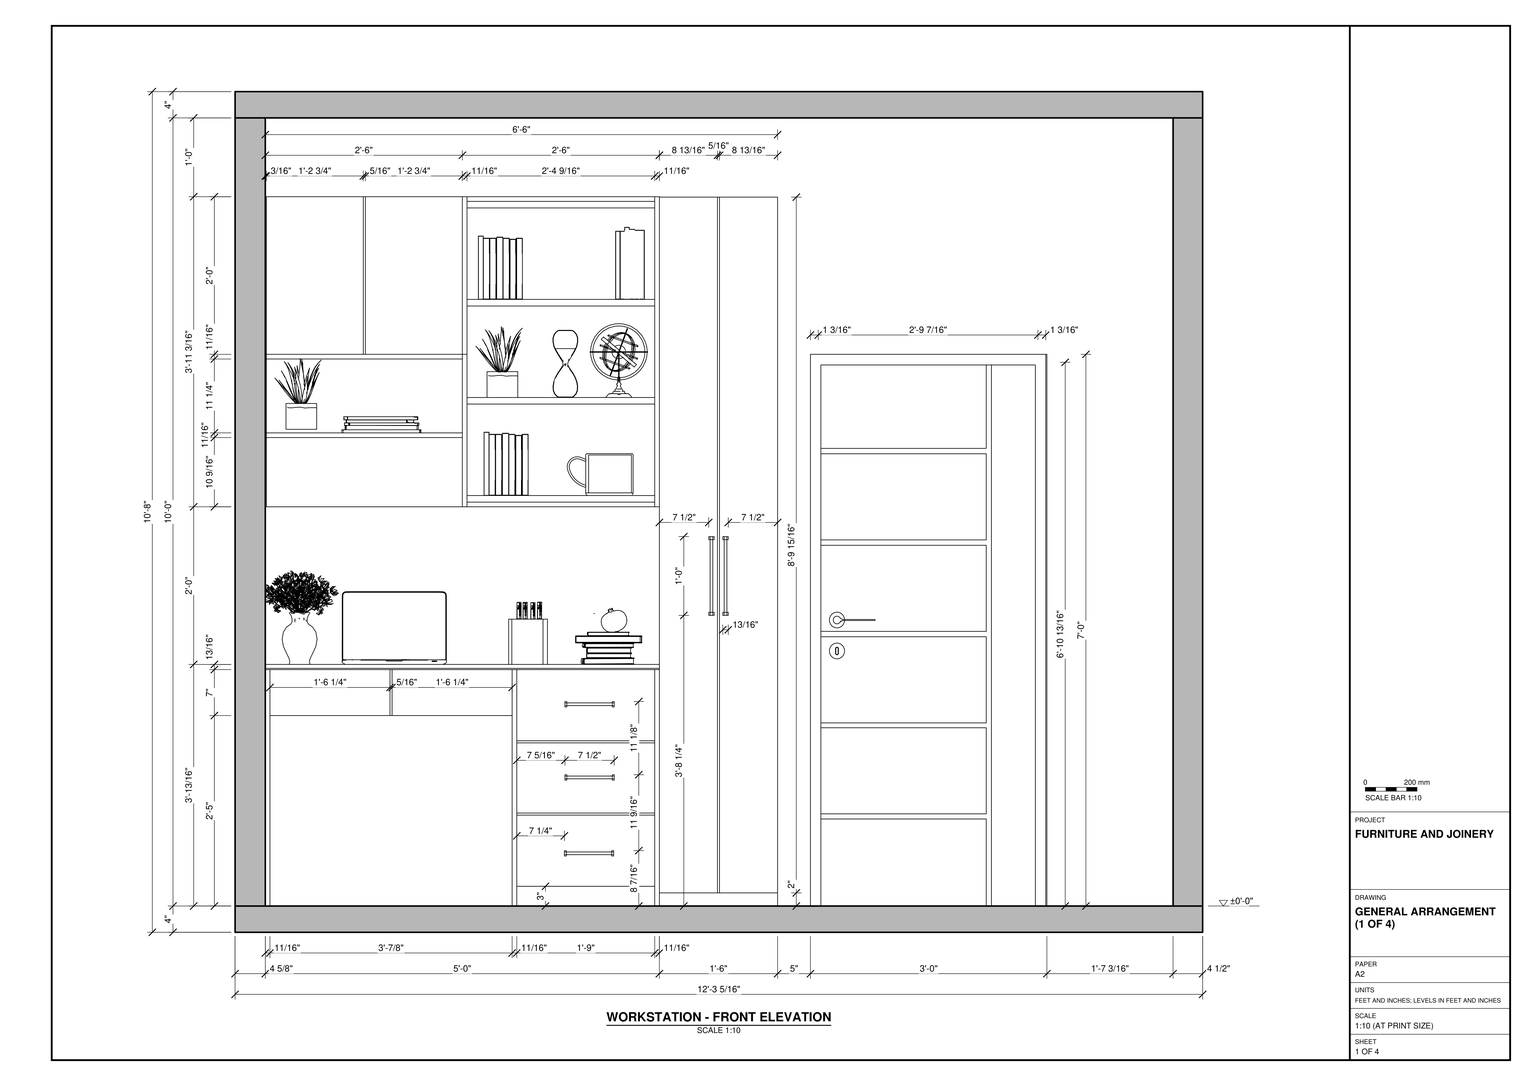
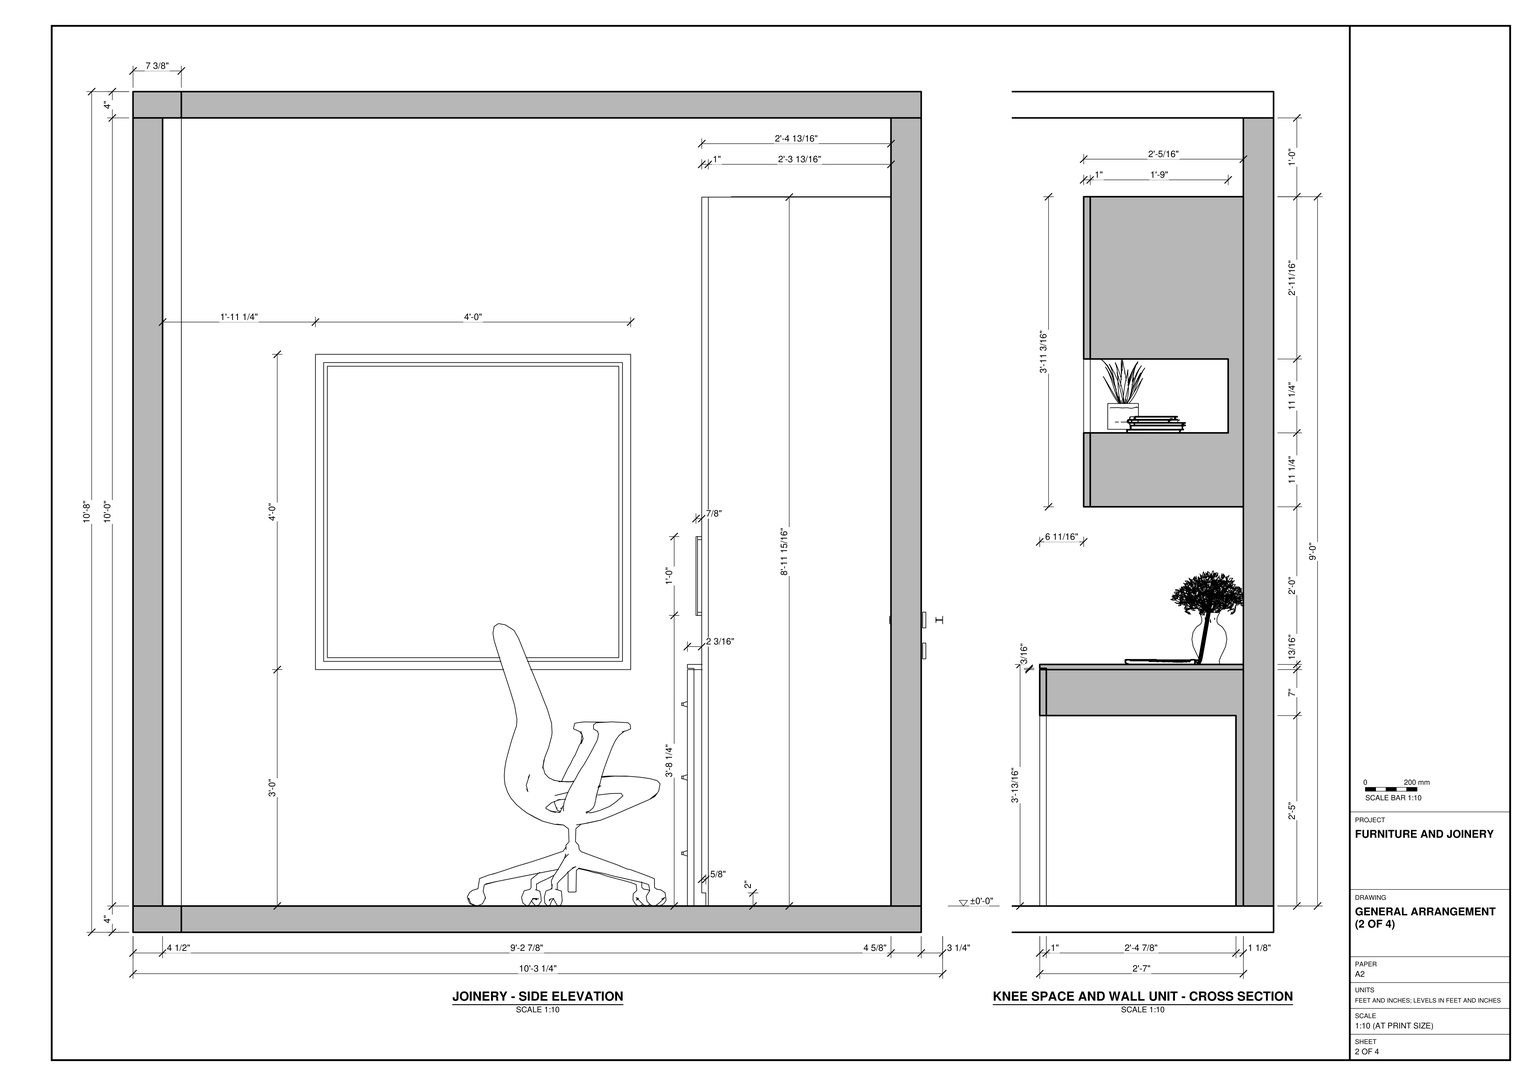
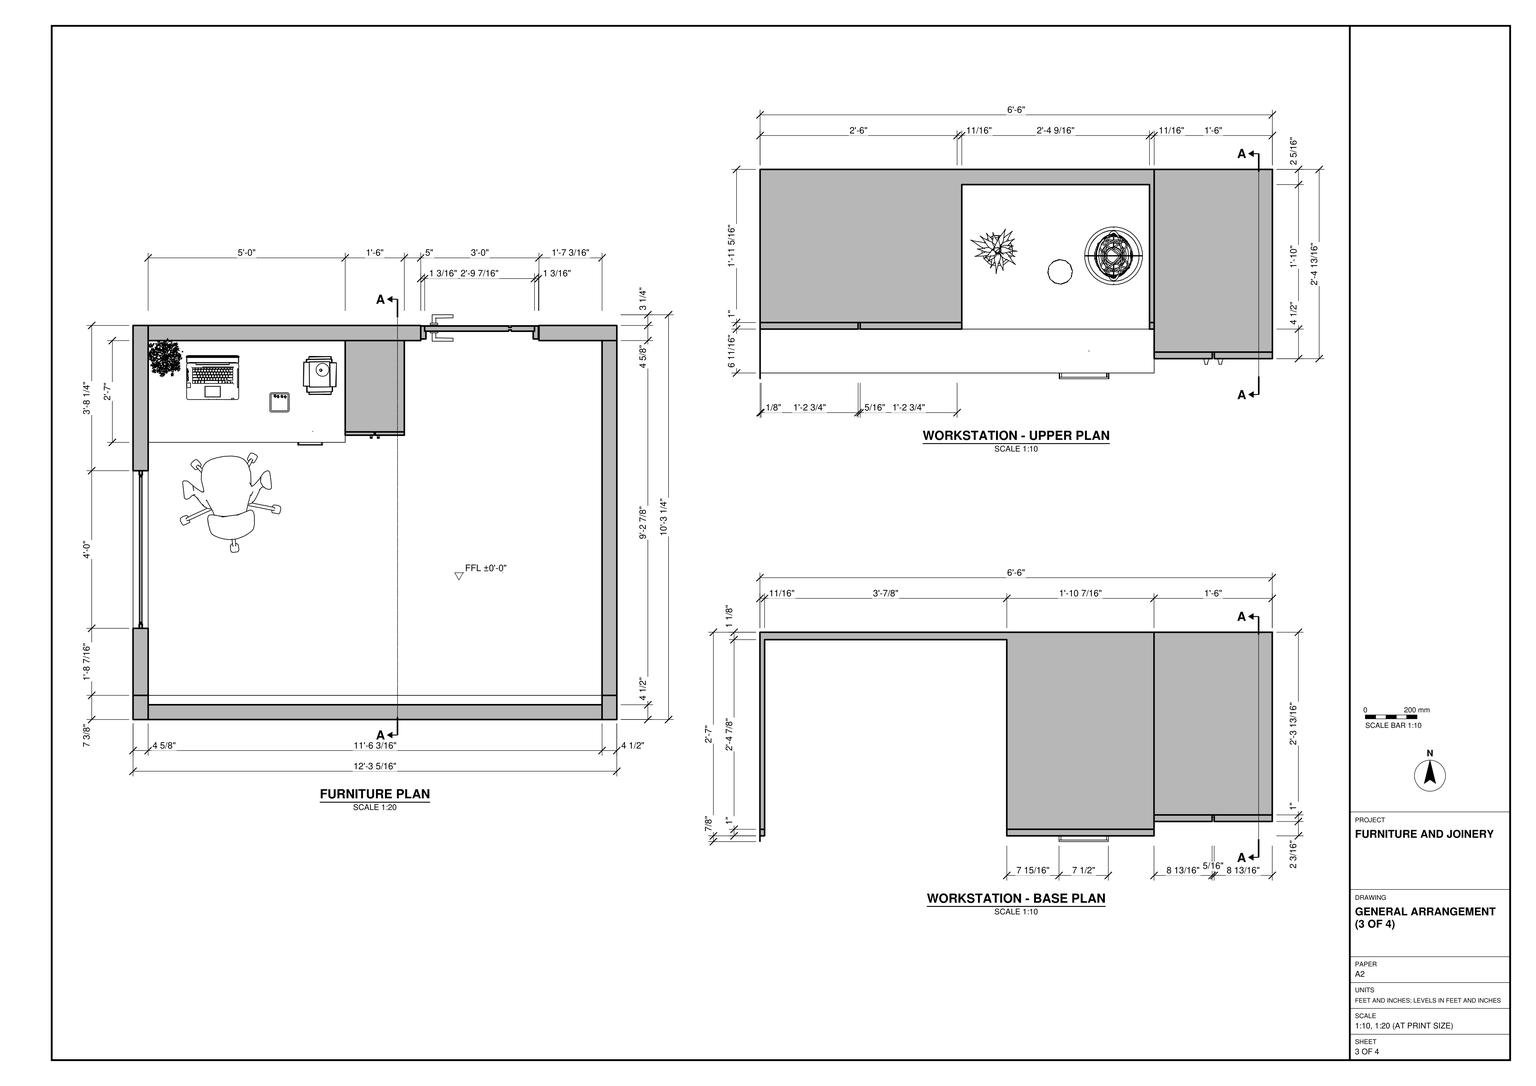
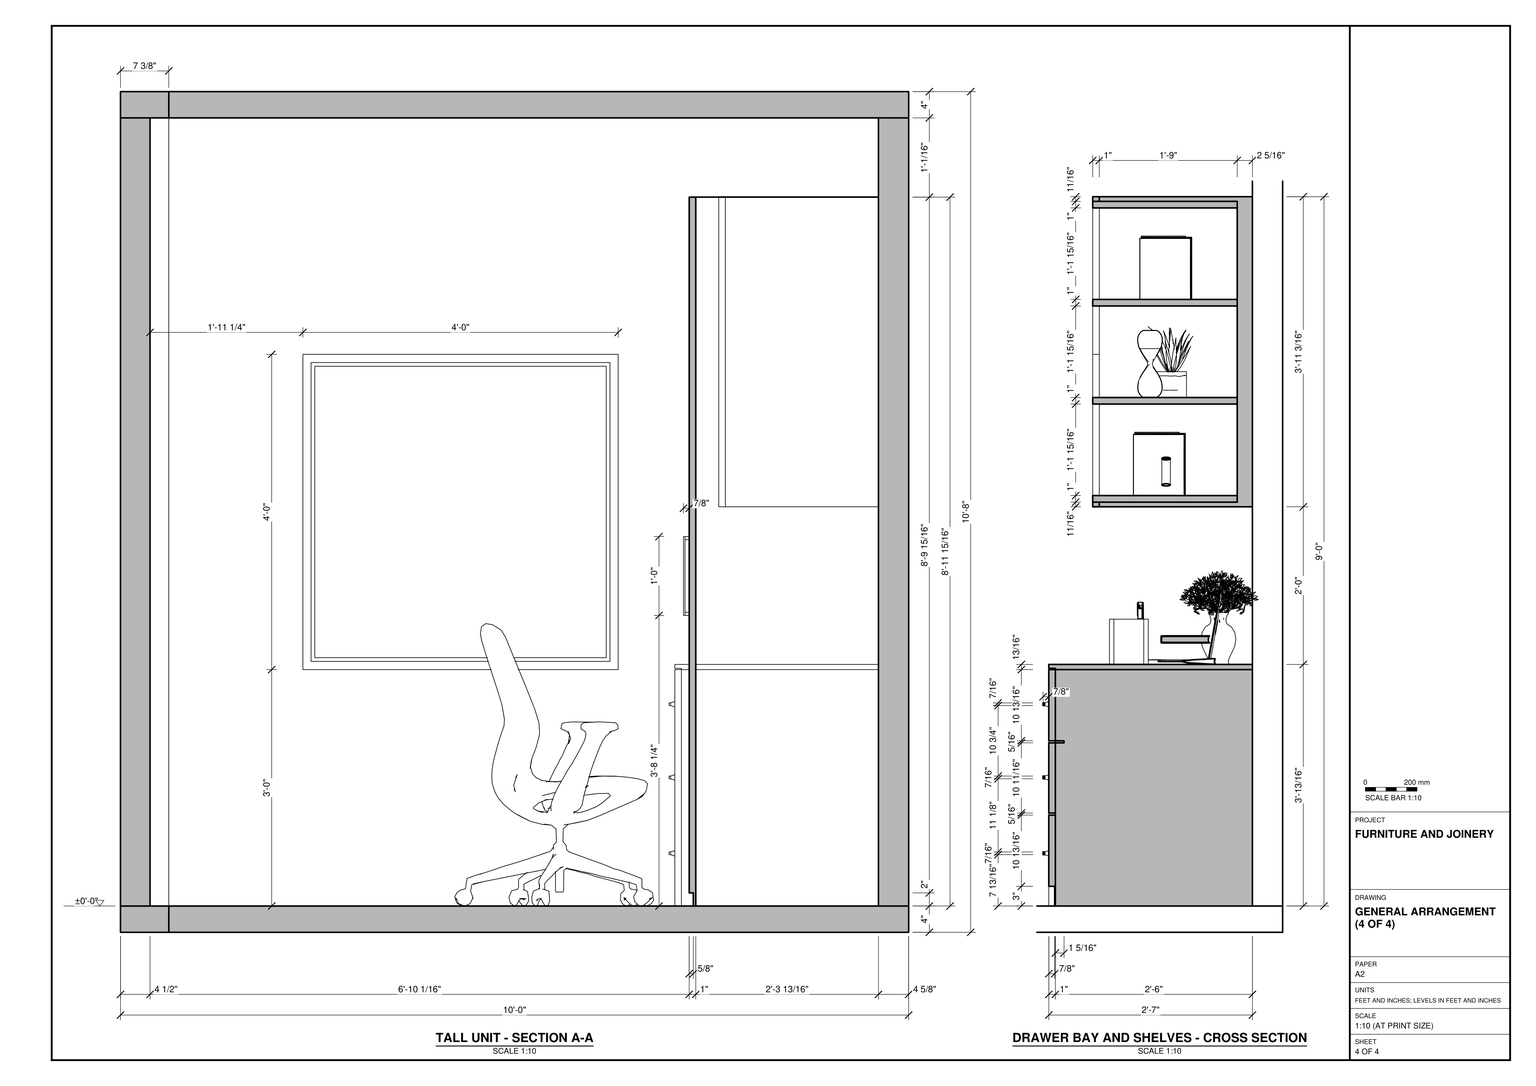
Work in feet and inches in SketchUp. Use task_files/diagram_01.pdf to model the room and its fitted workstation. The overall model measures 12'-3 5/16" along the workstation wall, 10'-3 1/4" in depth and 10'-8" in height. Set the finished floor at ±0'-0". Model the floor and ceiling slabs and follow the individual wall thicknesses in plan. Place the framed door to the right of the workstation and the square window in the adjoining left wall.

Build the workstation from the left corner toward the door. Use the base plan for the 5'-0" desk and its depth of 2'-7". Leave knee space beneath the shallow drawers and place the drawer pedestal to their right. Fit the tall paired-door cabinet between the desk and the doorway. Above the desk, reproduce the closed cupboards and open shelf bays, using the upper plan and cross section to set their depths and clearance above the worktop. Position the office chair facing the desk. Place the laptop, books, plants and desk accessories in the worktop and shelf locations shown. Decor and loose items may be any suitable library components.

Keep the walls, slabs and each furniture or joinery piece in separate groups or components, and use components for repeated parts. Save one SketchUp model as output_files/study_room_with_a_built_in_workstation.skp.

# SketchUp Ruby script. Lengths in inches.
U = 1.inch
M = Sketchup.active_model
def pt(a) = Geom::Point3d.new(a.map { |v| v * U })
def face(e, loops, mat)
  f = e.add_face(loops[0].map { |a| pt(a) })
  loops[1..].each { |l| e.add_face(l.map { |a| pt(a) }).erase! }
  f.material = f.back_material = mat if mat
  f
end
# faces: each face lists its corners as indices into pts; further lists are holes
def faces(e, pts, list, mat = nil) = list.each { |f| face(e, (f[0].is_a?(Array) ? f : [f]).map { |l| l.map { |i| pts[i] } }, mat) }
# xy, xz, yz: faces in a plane at the given z, y or x. An outline is a flat list of corners, or four numbers for a rectangle; further outlines are holes
def ring(l) = l.size == 4 ? [[l[0], l[1]], [l[2], l[1]], [l[2], l[3]], [l[0], l[3]]] : l.each_slice(2).to_a
def flat(e, list, mat, &to3) = list.each { |f| face(e, (f[0].is_a?(Array) ? f : [f]).map { |l| ring(l).map { |u, v| to3.(u, v) } }, mat) }
def xy(e, z, list, mat = nil) = flat(e, list, mat) { |x, y| [x, y, z] }
def xz(e, y, list, mat = nil) = flat(e, list, mat) { |x, z| [x, y, z] }
def yz(e, x, list, mat = nil) = flat(e, list, mat) { |y, z| [x, y, z] }
def lines(e, pts, list) = list.each { |a, b| e.add_line(pt(pts[a]), pt(pts[b])) }
# prism: a flat outline (further loops are holes) pulled along v
def prism(e, loops, v, mat = nil)
  f = face(e, loops, mat); d = Geom::Vector3d.new(v.map { |x| x * U })
  f.pushpull(f.normal.samedirection?(d) ? d.length : -d.length)
end
def box(e, o, s, mat = nil) = prism(e, [[o, [o[0] + s[0], o[1], o[2]], [o[0] + s[0], o[1] + s[1], o[2]], [o[0], o[1] + s[1], o[2]]]], [0, 0, s[2]], mat)
def at(x, y, z, deg = 0) = Geom::Transformation.translation(pt([x, y, z])) * Geom::Transformation.rotation(ORIGIN, Z_AXIS, deg.degrees)
def axes(o, x, y, z) = Geom::Transformation.new([*x, 0, *y, 0, *z, 0, *pt(o).to_a, 1])
def part(name) = M.definitions.add(name)
# library, detail: a bought-in or finely detailed component or shape, given as its bounding box
def library(name, o, s) = part(name).tap { |d| box(d.entities, o, s) }
def detail(e, o, s) = box(e.add_group.entities, o, s)
def put(e, d, t, mat = nil) = e.add_instance(d, t).tap { |i| i.material = mat if mat }
def group(e, t, mat = nil) = e.add_group.tap { |g| g.transformation = t; g.material = mat if mat }.entities
root = M.entities
M.materials.add("PVC Olive Green Matte 001").color = [133, 140, 86]
M.materials.add("Tiles Marble White 03 180cm").color = [241, 241, 241]
M.materials.add("Wood 021 27.52cm").color = [255, 255, 255]
c1 = part("POI-E1497-320-1917\#1")
xy(c1.entities,0,[[0,0,0.29,0.83],[7.21,0,7.5,0.83]])
xy(c1.entities,0.64,[[0.29,0.21,7.21,0.62]])
xy(c1.entities,0.875,[[0,0.21,7.5,0.62]])
xz(c1.entities,0.21,[[0,0.64,7.5,0.875]])
xz(c1.entities,0.62,[[0,0.64,7.5,0.875]])
yz(c1.entities,0,[[0,0,0.21,0.64,0.21,0.875,0.62,0.875,0.62,0.64,0.83,0]])
yz(c1.entities,0.29,[[0,0,0.83,0,0.62,0.64,0.21,0.64]])
yz(c1.entities,7.21,[[0,0,0.21,0.64,0.62,0.64,0.83,0]])
yz(c1.entities,7.5,[[0,0,0.83,0,0.62,0.64,0.62,0.875,0.21,0.875,0.21,0.64]])
p = [[0,0.21,0.64],[0,0,0],[0.29,0,0],[0.29,0.21,0.64],[7.21,0.21,0.64],[7.21,0,0],
  [7.5,0,0],[7.5,0.21,0.64],[0,0.83,0],[0,0.62,0.64],[0.29,0.62,0.64],[0.29,0.83,0],
  [7.5,0.83,0],[7.5,0.62,0.64],[7.21,0.62,0.64],[7.21,0.83,0]]
faces(c1.entities,p,[[0,1,2,3],[4,5,6,7],[8,9,10,11],[12,13,14,15]])
c2 = part("Group15\#1")
p = [[0,0,0],[0,0,-10.57],[-4.61,0,-10.57],[30,-4.22,0],[-30,-4.22,0],[30,4.22,0],
  [30,0,0],[-30,4.22,0],[4.61,0,-10.57],[-30,0,0],[0,0,-17.11]]
lines(c2.entities,p,[[0,1],[1,2],[3,4],[5,6],[7,5],[1,8],[9,0],[0,6],[8,10],[4,9],[6,3],[2,10],
  [9,7]])
c3 = part("Rectangle Light")
put(c3.entities,c2,at(0,0,0))
c4 = part("Group17\#1")
p = [[0,0,0],[0,0,-5.7],[-2.29,0,-5.7],[14.92,-3.53,0],[-14.92,-3.53,0],[14.92,3.53,0],
  [14.92,0,0],[-14.92,3.53,0],[2.29,0,-5.7],[-14.92,0,0],[0,0,-9.23]]
lines(c4.entities,p,[[0,1],[1,2],[3,4],[5,6],[7,5],[1,8],[9,0],[0,6],[8,10],[4,9],[6,3],[2,10],
  [9,7]])
c5 = part("Rectangle Light\#1")
put(c5.entities,c4,at(0,0,0))
c6 = part("Group19\#1")
p = [[0,0,0],[0,0,-5.18],[-2.2,0,-5.18],[14.29,-2.48,0],[-14.29,-2.48,0],[14.29,2.48,0],
  [14.29,0,0],[-14.29,2.48,0],[2.2,0,-5.18],[-14.29,0,0],[0,0,-8.39]]
lines(c6.entities,p,[[0,1],[1,2],[3,4],[5,6],[7,5],[1,8],[9,0],[0,6],[8,10],[4,9],[6,3],[2,10],
  [9,7]])
c7 = part("Rectangle Light\#2")
put(c7.entities,c6,at(0,0,0))
c8 = part("Group21\#1")
p = [[0,0,0],[0,0,-5.25],[-2.2,0,-5.25],[14.29,-2.69,0],[-14.29,-2.69,0],[14.29,2.69,0],
  [14.29,0,0],[-14.29,2.69,0],[2.2,0,-5.25],[-14.29,0,0],[0,0,-8.49]]
lines(c8.entities,p,[[0,1],[1,2],[3,4],[5,6],[7,5],[1,8],[9,0],[0,6],[8,10],[4,9],[6,3],[2,10],
  [9,7]])
c9 = part("Rectangle Light\#3")
put(c9.entities,c8,at(0,0,0))
c10 = part("Group23\#1")
p = [[0,0,0],[0,0,-5.4],[-2.2,0,-5.4],[14.29,-3.19,0],[-14.29,-3.19,0],[14.29,3.19,0],
  [14.29,0,0],[-14.29,3.19,0],[2.2,0,-5.4],[-14.29,0,0],[0,0,-8.74]]
lines(c10.entities,p,[[0,1],[1,2],[3,4],[5,6],[7,5],[1,8],[9,0],[0,6],[8,10],[4,9],[6,3],[2,10],
  [9,7]])
c11 = part("Rectangle Light\#4")
put(c11.entities,c10,at(0,0,0))
c12 = library("Laptop 013",[-7.94,-6.65,0],[15.87,13.3,11.09])
c13 = library("Vase Flowers 26-02",[-5.76,-5.9,0],[11.73,12.02,14.27])
c14 = library("Books 155 025",[-5.0625,-5.83,0.01],[10.11,11.66,8.59])
c15 = library("Books 53-13",[-3.36,-3.97,0],[6.72,7.94,9.65])
c16 = library("Books 53-17",[-2.19,-3.6875,0],[4.38,7.37,10.99])
c17 = library("pen_stand",[0,-5.91,0],[13.07,11.82,9.49])
c18 = library("Books 193 003",[-6.07,-4.15,0],[12.06,9.04,2.47])
c19 = library("Potted Succulent 003",[-4.09,-3.62,0],[7.1,6.83,10.79])
c20 = library("Decorative Hourglass 001",[-1.06,-1.06,0.02],[2.12,2.12,5.71])
c21 = library("Armillary Sphere 37-31",[-7.11,-7.1,0],[14.21,14.18,18.13])
c22 = library("Chair 233 035",[-15.42,-13.39,-0.11],[30.84,29.38,43.01])
c23 = library("PINTU 6 YA",[0,-0.6875,0],[35.83,8.07,80.71])
c24 = library("Group\#29",[0,0,0],[5.48,3.93,3.49])
c25 = part("Group88\#1")
xz(c25.entities,32.25,[[29.52,0,176.83,4]])
c26 = part("Group90\#1")
xz(c26.entities,32.25,[[29.52,4,34.12,124]])
c27 = part("Group188\#1")
xz(c27.entities,32.25,[[172.33,4,176.83,124]])
c28 = part("Group218\#1")
xz(c28.entities,32.25,[[29.52,124,176.83,128]])
c29 = part("Group83\#1")
put(c29.entities,c25,at(0,0,0))
put(c29.entities,c26,at(0,0,0))
put(c29.entities,c27,at(0,0,0))
put(c29.entities,c28,at(0,0,0))
p = [[2.3,75.77,40],[2.3,27.77,40],[2.3,27.77,88],[2.3,75.77,88]]
lines(root,p,[[0,1],[1,2],[2,3],[3,0]])
put(root,c1,axes([57.72,84.4,34.31],[-1,0,0],[0,0,1],[0,-1,0]))
put(root,c1,axes([57.72,84.4,23.17],[-1,0,0],[0,0,1],[0,-1,0]))
put(root,c1,axes([57.64,84.4,11.61],[-1,0,0],[0,0,1],[0,-1,0]))
put(root,c1,axes([72.11,86.59,48.25],[0,0,1.6],[1,0,0],[0,-1,0]))
put(root,c1,axes([74.26,86.59,48.25],[0,0,1.6],[1,0,0],[0,-1,0]))
put(root,c3,axes([34.6,111.18,64.78],[1,0,0],[0,-1,0],[0,0,0.21]))
put(root,c5,axes([19.68,109.56,87.28],[1,0,0],[0,-1,0],[0,0,0.2]))
put(root,c7,axes([49.6,110.61,110.28],[1,0,0],[0,-1,0],[0,0,0.32]))
put(root,c9,axes([49.6,110.39,95.35],[1,0,0],[0,-1,0],[0,0,0.28]))
put(root,c11,axes([49.6,109.9,80.42],[1,0,0],[0,-1,0],[0,0,0.33]))
put(root,c12,at(24.24,104.09,40.79))
put(root,c13,at(9.83,110.23,40.79))
put(root,c14,at(56.89,104.76,40.77))
put(root,c15,at(41.26,101.23,66.5))
put(root,c15,at(40.39,102.21,96.36))
put(root,c16,at(60.125,101.11,96.36))
put(root,c17,at(41.65,93.64,40.79))
put(root,c18,at(22.32,101.81,76.04))
put(root,c19,at(10.13,97.19,76.58))
put(root,c20,axes([50.28,99.8,81.41],[1.79,0,0],[0,1.79,0],[0,0,1.79]))
put(root,c21,axes([58.43,102.25,81.43],[0.62,0,0],[0,0.62,0],[0,0,0.62]))
put(root,c19,at(40.74,103.13,81.43))
put(root,c22,at(29.17,66.85,4.11,-173.2))
put(root,c23,axes([87.6,115.89,4],[1,0,0],[0,1,0],[0,0,1.04078]))
g1 = group(root,at(0,0,0))
xy(g1,0,[[0,0,147.3125,120]])
xy(g1,4,[[0,0,147.3125,120]],"Tiles Marble White 03 180cm")
xz(g1,0,[[0,0,147.3125,4]])
xz(g1,120,[[0,0,147.3125,4]])
yz(g1,0,[[0,0,120,4]])
yz(g1,147.3125,[[0,0,120,4]])
g2 = group(root,at(0,0,4))
xy(g2,0,[[0,0,4.6,120]])
xy(g2,36,[[0,27.77,4.6,75.77]])
xy(g2,84,[[0,27.77,4.6,75.77]])
xy(g2,120,[[0,0,4.6,120]])
xz(g2,0,[[0,0,4.6,120]])
xz(g2,27.77,[[0,36,4.6,84]])
xz(g2,75.77,[[0,36,4.6,84]])
xz(g2,120,[[0,0,4.6,120]])
yz(g2,0,[[[0,0,120,120],[27.77,36,75.77,84]]])
yz(g2,4.6,[[[0,0,115.4,120],[27.77,36,75.77,84]],[115.4,0,120,120]])
g3 = group(root,at(4.6,115.4,4))
prism(g3,[[[142.71,4.6,0],[119,4.6,0],[119,4.6,84],[83,4.6,84],[83,4.6,0],[0,4.6,0],[0,4.6,120],[142.71,4.6,120]]],[0,-4.6,0])
g4 = group(root,at(4.6,85.4,4))
xy(g4,0,[[0,0,0,30,60,30,60,0,37.58,0,37.58,28.875,0.71,28.875,0.71,0]])
xy(g4,29,[[0.71,0,37.58,28.875]])
xy(g4,36,[[0,0,60,30]])
xz(g4,0,[[0,0,0.71,0,0.71,29,37.58,29,37.58,0,60,0,60,36,0,36]])
xz(g4,28.875,[[0.71,0,37.58,29]])
xz(g4,30,[[0,0,60,36]])
yz(g4,0,[[0,0,30,36]])
yz(g4,0.71,[[0,0,28.875,29]])
yz(g4,37.58,[[0,0,28.875,29]])
yz(g4,60,[[0,0,30,36]])
g5 = group(root,at(4.6,84.4,4))
xy(g5,0,[[0,0,0.71,1],[37.58,0,37.58,1,60,1,60,0,59.29,0,59.29,0.9,38.29,0.9,38.29,0]])
xy(g5,3,[[38.29,0,59.29,0.9]])
xy(g5,13.84,[[38.29,0,59.29,1]])
xy(g5,14.16,[[38.29,0,59.29,1]])
xy(g5,24.84,[[38.29,0,59.29,2.3125]])
xy(g5,25.16,[[38.29,0,59.29,2.3125]])
xy(g5,29,[[0.71,0,18.99,1],[19.3,0,37.58,1]])
xy(g5,36,[[0,0,18.99,1],[19.3,0,60,1]])
xz(g5,0,[[0,0,0.71,36],[37.58,0,38.29,36],[59.29,0,60,36]])
xz(g5,0,[[38.29,3,59.29,13.84],[38.29,14.16,59.29,24.84],[38.29,25.16,59.29,36],[0.71,29,18.99,36],[19.3,29,37.58,36]],"PVC Olive Green Matte 001")
xz(g5,0.9,[[38.29,0,59.29,3]])
xz(g5,1,[[0,0,0,36,18.99,36,18.99,29,0.71,29,0.71,0],[[37.58,0,37.58,29,19.3,29,19.3,36,60,36,60,0],[38.29,13.84,59.29,14.16]],[18.99,29,19.3,36]])
xz(g5,2.3125,[[38.29,24.84,59.29,25.16]])
yz(g5,0,[[0,0,1,36]])
yz(g5,0.71,[[0,0,1,29]])
yz(g5,18.99,[[0,29,1,36]])
yz(g5,19.3,[[0,29,1,36]])
yz(g5,37.58,[[0,0,1,29]])
yz(g5,38.29,[[0,0,0.9,3],[0,13.84,1,14.16],[0,24.84,2.3125,25.16]])
yz(g5,59.29,[[0,0,0.9,3],[0,13.84,1,14.16],[0,24.84,2.3125,25.16]])
yz(g5,60,[[0,0,1,36]])
g6 = group(root,at(4.6,84.4,40))
prism(g6,[[[0,31,0],[0,1,0],[0,1,0.1875],[0,0,0.1875],[0,0,0.79],[0,31,0.79]]],[60,0,0],"PVC Olive Green Matte 001")
g7 = group(root,at(64.6,85.4,4))
box(g7,[0,2.1875,0],[18,27.8125,107.9375],"PVC Olive Green Matte 001")
g8 = group(root,at(64.6,86.59,4))
xy(g8,0,[[0,0.625,18,1]])
xy(g8,2,[[0,0,8.84,0.625],[9.16,0,18,0.625],[8.84,0.625,9.16,1]])
xy(g8,107.9375,[[0,0,8.84,1],[9.16,0,18,1]])
xz(g8,0,[[0,2,8.84,107.9375],[9.16,2,18,107.9375]],"PVC Olive Green Matte 001")
xz(g8,0.625,[[0,0,18,2]])
xz(g8,1,[[0,0,0,107.9375,8.84,107.9375,8.84,2,9.16,2,9.16,107.9375,18,107.9375,18,0]])
yz(g8,0,[[0.625,0,0.625,2,0,2,0,107.9375,1,107.9375,1,0]])
yz(g8,8.84,[[0,2,1,107.9375]])
yz(g8,9.16,[[0,2,1,107.9375]])
yz(g8,18,[[0.625,0,1,0,1,107.9375,0,107.9375,0,2,0.625,2]])
g9 = group(root,at(4.6,92.09,64.79))
xy(g9,0,[[0,0,60,23.3125]])
xy(g9,0.71,[[30.71,0,59.29,21]])
xy(g9,11.25,[[0.16,0,30,21]],"Wood 021 27.52cm")
xy(g9,22.5,[[0.16,0,30,21]])
xy(g9,46.5,[[30.71,0,59.29,21]])
xy(g9,47.21,[[0,0,60,23.3125]],"PVC Olive Green Matte 001")
xz(g9,0,[[[0,0,60,47.21],[30.71,0.71,59.29,46.5],[0.16,11.25,30,22.5]]])
xz(g9,21,[[30.71,0.71,59.29,46.5]])
xz(g9,21,[[0.16,11.25,30,22.5]],"Wood 021 27.52cm")
xz(g9,23.3125,[[0,0,60,47.21]])
yz(g9,0,[[0,0,23.3125,47.21]])
yz(g9,0.16,[[0,11.25,21,22.5]],"Wood 021 27.52cm")
yz(g9,30,[[0,11.25,21,22.5]],"Wood 021 27.52cm")
yz(g9,30.71,[[0,0.71,21,46.5]],"Wood 021 27.52cm")
yz(g9,59.29,[[0,0.71,21,46.5]],"Wood 021 27.52cm")
yz(g9,60,[[0,0,23.3125,47.21]])
g10 = group(root,at(4.6,91.09,64.79))
xy(g10,0,[[0,0,60,1]],"PVC Olive Green Matte 001")
xy(g10,0.71,[[30.71,0,59.29,1]],"PVC Olive Green Matte 001")
xy(g10,11.25,[[0.16,0,30,1]],"PVC Olive Green Matte 001")
xy(g10,22.5,[[0.16,0,30,1]],"PVC Olive Green Matte 001")
xy(g10,23.21,[[14.92,0,15.24,1]],"PVC Olive Green Matte 001")
xy(g10,46.5,[[30.71,0,59.29,1]],"PVC Olive Green Matte 001")
xy(g10,47.21,[[0,0,14.92,1],[15.24,0,60,1]],"PVC Olive Green Matte 001")
xz(g10,0,[[0,0,0.16,10.54],[0.16,0,30,10.54],[30,0,30.71,23.21],[30.71,0,59.29,0.71],[59.29,0,60,47.21],
  [0,10.54,0.16,11.25],[0.16,10.54,30,11.25],[0,11.25,0.16,22.5],[0,22.5,0.16,23.21],[0.16,22.5,30,23.21],
  [0,23.21,0.16,47.21],[0.16,23.21,14.92,47.21],[15.24,23.21,30,47.21],[30,23.21,30.71,47.21],[30.71,46.5,59.29,47.21]],"PVC Olive Green Matte 001")
xz(g10,1,[[[0,0,0,47.21,14.92,47.21,14.92,23.21,15.24,23.21,15.24,47.21,60,47.21,60,0],[30.71,0.71,59.29,46.5],[0.16,11.25,30,22.5]]],"PVC Olive Green Matte 001")
yz(g10,0,[[0,0,1,47.21]],"PVC Olive Green Matte 001")
yz(g10,0.16,[[0,11.25,1,22.5]],"PVC Olive Green Matte 001")
yz(g10,14.92,[[0,23.21,1,47.21]],"PVC Olive Green Matte 001")
yz(g10,15.24,[[0,23.21,1,47.21]],"PVC Olive Green Matte 001")
yz(g10,30,[[0,11.25,1,22.5]],"PVC Olive Green Matte 001")
yz(g10,30.71,[[0,0.71,1,23.21],[0,23.21,1,46.5]],"PVC Olive Green Matte 001")
yz(g10,59.29,[[0,0.71,1,46.5]],"PVC Olive Green Matte 001")
yz(g10,60,[[0,0,1,47.21]],"PVC Olive Green Matte 001")
g11 = group(root,at(35.31,91.09,65.5))
xy(g11,0,[[0,0,28.58,22]])
xy(g11,1,[[0,0,28.58,22]],"Wood 021 27.52cm")
xz(g11,0,[[0,0,28.58,1]])
xz(g11,22,[[0,0,28.58,1]])
yz(g11,0,[[0,0,22,1]])
yz(g11,28.58,[[0,0,22,1]])
g12 = group(root,at(35.31,91.09,80.43))
box(g12,[0,0,0],[28.58,22,1],"Wood 021 27.52cm")
g13 = group(root,at(35.31,91.09,95.36),"Wood 021 27.52cm")
xy(g13,0,[[0,0,28.58,22]])
xy(g13,1,[[0,0,28.58,22]])
xz(g13,0,[[0,0,28.58,1]],"Wood 021 27.52cm")
xz(g13,22,[[0,0,28.58,1]])
yz(g13,0,[[0,0,22,1]])
yz(g13,28.58,[[0,0,22,1]])
g14 = group(root,at(35.31,91.09,110.29))
xy(g14,0,[[0,0,28.58,22]],"Wood 021 27.52cm")
xy(g14,1,[[0,0,28.58,22]])
xz(g14,0,[[0,0,28.58,1]],"Wood 021 27.52cm")
xz(g14,22,[[0,0,28.58,1]])
yz(g14,0,[[0,0,22,1]])
yz(g14,28.58,[[0,0,22,1]])
g15 = group(root,at(1.875,27.77,40))
xy(g15,0,[[0,0,0.9375,48]])
xy(g15,1.25,[[0,1.25,0.22,46.75],[0.66,1.25,0.9375,46.75]])
xy(g15,1.8125,[[0.22,1.8125,0.66,46.1875]])
xy(g15,46.1875,[[0.22,1.8125,0.66,46.1875]])
xy(g15,46.75,[[0,1.25,0.22,46.75],[0.66,1.25,0.9375,46.75]])
xy(g15,48,[[0,0,0.9375,48]])
xz(g15,0,[[0,0,0.9375,48]])
xz(g15,1.25,[[0,1.25,0.22,46.75],[0.66,1.25,0.9375,46.75]])
xz(g15,1.8125,[[0.22,1.8125,0.66,46.1875]])
xz(g15,46.1875,[[0.22,1.8125,0.66,46.1875]])
xz(g15,46.75,[[0,1.25,0.22,46.75],[0.66,1.25,0.9375,46.75]])
xz(g15,48,[[0,0,0.9375,48]])
yz(g15,0,[[[0,0,48,48],[1.25,1.25,46.75,46.75]]])
yz(g15,0.22,[[[1.25,1.25,46.75,46.75],[1.8125,1.8125,46.1875,46.1875]]])
yz(g15,0.66,[[[1.25,1.25,46.75,46.75],[1.8125,1.8125,46.1875,46.1875]]])
yz(g15,0.9375,[[[0,0,48,48],[1.25,1.25,46.75,46.75]]])
put(root,c24,axes([50.57,98.51,66.5],[1.83,0,0],[0,1.83,0],[0,0,1.83]))
g16 = group(root,at(142.8125,0,4))
box(g16,[0,0,0],[4.5,115.4,120])
g17 = group(root,at(4.6,0,4))
box(g17,[0,0,0],[138.21,4.5,120])
g18 = group(root,at(0,0,124))
box(g18,[0,0,0],[147.3125,120,4])
put(root,c29,at(-29.52,-24.89,0))
